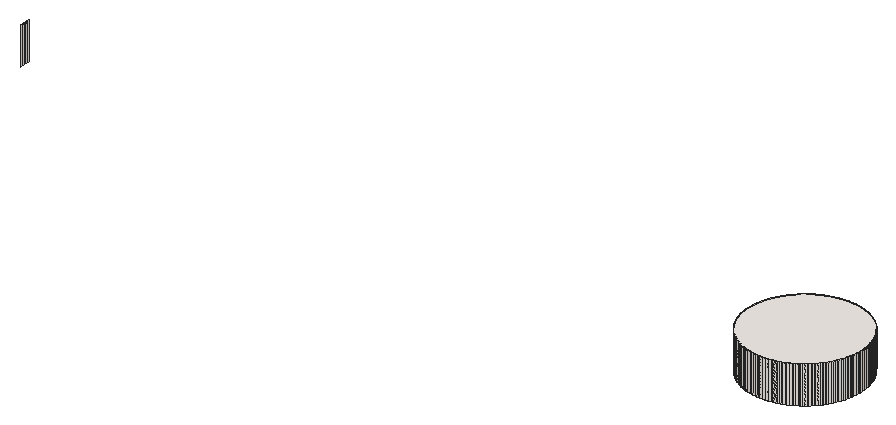
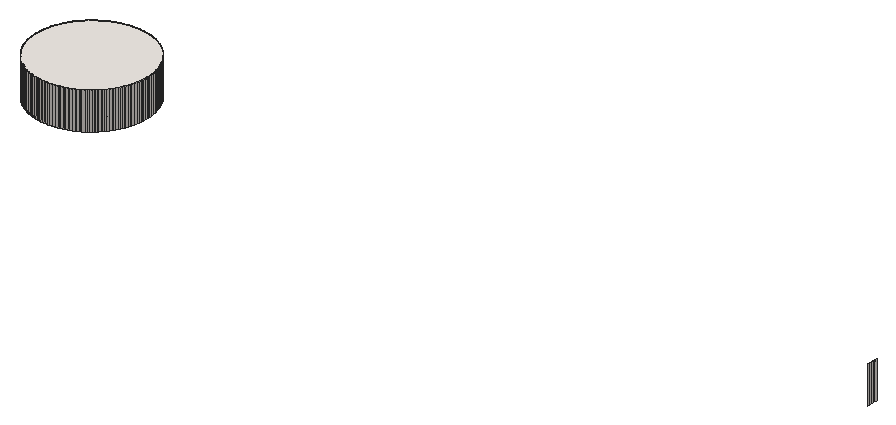
# SketchUp Ruby script. Lengths in inches.
U = 1.inch
M = Sketchup.active_model
def pt(a) = Geom::Point3d.new(a.map { |v| v * U })
def face(e, loops, mat)
  f = e.add_face(loops[0].map { |a| pt(a) })
  loops[1..].each { |l| e.add_face(l.map { |a| pt(a) }).erase! }
  f.material = f.back_material = mat if mat
  f
end
# faces: each face lists its corners as indices into pts; further lists are holes
def faces(e, pts, list, mat = nil) = list.each { |f| face(e, (f[0].is_a?(Array) ? f : [f]).map { |l| l.map { |i| pts[i] } }, mat) }
# xy, xz, yz: faces in a plane at the given z, y or x. An outline is a flat list of corners, or four numbers for a rectangle; further outlines are holes
def ring(l) = l.size == 4 ? [[l[0], l[1]], [l[2], l[1]], [l[2], l[3]], [l[0], l[3]]] : l.each_slice(2).to_a
def flat(e, list, mat, &to3) = list.each { |f| face(e, (f[0].is_a?(Array) ? f : [f]).map { |l| ring(l).map { |u, v| to3.(u, v) } }, mat) }
def xy(e, z, list, mat = nil) = flat(e, list, mat) { |x, y| [x, y, z] }
def xz(e, y, list, mat = nil) = flat(e, list, mat) { |x, z| [x, y, z] }
def yz(e, x, list, mat = nil) = flat(e, list, mat) { |y, z| [x, y, z] }
def lines(e, pts, list) = list.each { |a, b| e.add_line(pt(pts[a]), pt(pts[b])) }
# prism: a flat outline (further loops are holes) pulled along v
def prism(e, loops, v, mat = nil)
  f = face(e, loops, mat); d = Geom::Vector3d.new(v.map { |x| x * U })
  f.pushpull(f.normal.samedirection?(d) ? d.length : -d.length)
end
def box(e, o, s, mat = nil) = prism(e, [[o, [o[0] + s[0], o[1], o[2]], [o[0] + s[0], o[1] + s[1], o[2]], [o[0], o[1] + s[1], o[2]]]], [0, 0, s[2]], mat)
def at(x, y, z, deg = 0) = Geom::Transformation.translation(pt([x, y, z])) * Geom::Transformation.rotation(ORIGIN, Z_AXIS, deg.degrees)
def axes(o, x, y, z) = Geom::Transformation.new([*x, 0, *y, 0, *z, 0, *pt(o).to_a, 1])
def part(name) = M.definitions.add(name)
# library, detail: a bought-in or finely detailed component or shape, given as its bounding box
def library(name, o, s) = part(name).tap { |d| box(d.entities, o, s) }
def detail(e, o, s) = box(e.add_group.entities, o, s)
def put(e, d, t, mat = nil) = e.add_instance(d, t).tap { |i| i.material = mat if mat }
def group(e, t, mat = nil) = e.add_group.tap { |g| g.transformation = t; g.material = mat if mat }.entities
root = M.entities
M.materials.add("0001 AP 9436 AIR BREEZE").color = [243, 237, 232]
xy(root,108,[[158.91,40.5,158.83,40.51,158.75,40.51,158.51,40.54,158.4375,40.55,158.36,40.57,158.28,40.59,158.21,40.61,158.13,40.63,158.06,40.65,157.98,40.68,157.91,40.71,157.84,40.73,157.76,40.77,157.69,40.8,157.625,40.83,157.55,40.87,157.49,40.91,157.35,40.99,157.29,41.04,157.22,41.08,156.98,41.28,156.87,41.39,156.8125,41.45,156.76,41.5,156.61,41.6875,156.5625,41.75,156.52,41.8125,156.48,41.88,156.43,41.95,156.39,42.01,156.36,42.08,156.32,42.15,156.29,42.22,156.25,42.29,156.22,42.37,156.19,42.44,156.17,42.51,156.14,42.59,156.12,42.66,156.0625,42.89,156.05,42.97,156.03,43.05,156.01,43.2,156.01,43.28,156,43.36,156,43.59,156.01,43.67,156.01,43.75,156.04,43.99,156.05,44.0625,156.07,44.14,156.09,44.22,156.11,44.29,156.13,44.37,156.15,44.44,156.18,44.52,156.21,44.59,156.23,44.66,156.27,44.74,156.3,44.81,156.33,44.875,156.37,44.95,156.41,45.01,156.49,45.15,156.54,45.21,156.58,45.28,156.78,45.52,156.89,45.63,156.95,45.6875,157,45.74,157.1875,45.89,157.25,45.9375,157.3125,45.98,157.38,46.02,157.45,46.07,157.51,46.11,157.58,46.14,157.65,46.18,157.72,46.21,157.79,46.25,157.87,46.28,157.94,46.31,158.01,46.33,158.09,46.36,158.16,46.38,158.39,46.4375,158.47,46.45,158.55,46.47,158.7,46.49,158.78,46.49,158.86,46.5,159.09,46.5,159.17,46.49,159.25,46.49,159.49,46.46,159.5625,46.45,159.64,46.43,159.72,46.41,159.79,46.39,159.87,46.37,159.94,46.35,160.02,46.32,160.09,46.29,160.16,46.27,160.24,46.23,160.31,46.2,160.375,46.17,160.45,46.13,160.51,46.09,160.65,46.01,160.71,45.96,160.78,45.92,161.02,45.72,161.13,45.61,161.1875,45.55,161.24,45.5,161.39,45.3125,161.4375,45.25,161.48,45.1875,161.52,45.12,161.57,45.05,161.61,44.99,161.64,44.92,161.68,44.85,161.71,44.78,161.75,44.71,161.78,44.63,161.81,44.56,161.83,44.49,161.86,44.41,161.88,44.34,161.9375,44.11,161.95,44.03,161.97,43.95,161.99,43.8,161.99,43.72,162,43.64,162,43.41,161.99,43.33,161.99,43.25,161.96,43.01,161.95,42.9375,161.93,42.86,161.91,42.78,161.89,42.71,161.87,42.63,161.85,42.56,161.82,42.48,161.79,42.41,161.77,42.34,161.73,42.26,161.7,42.19,161.67,42.125,161.63,42.05,161.59,41.99,161.51,41.85,161.46,41.79,161.42,41.72,161.22,41.48,161.11,41.37,161.05,41.3125,161,41.26,160.8125,41.11,160.75,41.0625,160.6875,41.02,160.62,40.98,160.55,40.93,160.49,40.89,160.42,40.86,160.35,40.82,160.28,40.79,160.21,40.75,160.13,40.72,160.06,40.69,159.99,40.67,159.91,40.64,159.84,40.62,159.61,40.5625,159.53,40.55,159.45,40.53,159.3,40.51,159.22,40.51,159.14,40.5]],"0001 AP 9436 AIR BREEZE")
xz(root,40.5,[[158.91,106,158.98,108],[158.98,106,159.0625,108],[159.0625,106,159.14,108]],"0001 AP 9436 AIR BREEZE")
xz(root,40.51,[[158.75,106,158.83,108],[159.22,106,159.3,108]],"0001 AP 9436 AIR BREEZE")
xz(root,46.49,[[158.7,106,158.78,108],[159.17,106,159.25,108]],"0001 AP 9436 AIR BREEZE")
xz(root,46.5,[[158.86,106,158.9375,108],[158.9375,106,159.02,108],[159.02,106,159.09,108]],"0001 AP 9436 AIR BREEZE")
yz(root,116.99,[[43.25,106,43.33,108],[43.72,106,43.8,108]],"0001 AP 9436 AIR BREEZE")
yz(root,117,[[43.41,106,43.48,108],[43.48,106,43.5625,108],[43.5625,106,43.64,108]],"0001 AP 9436 AIR BREEZE")
yz(root,156,[[43.36,106,43.4375,108],[43.4375,106,43.52,108],[43.52,106,43.59,108]],"0001 AP 9436 AIR BREEZE")
yz(root,156.01,[[43.2,106,43.28,108],[43.67,106,43.75,108]],"0001 AP 9436 AIR BREEZE")
yz(root,161.99,[[43.25,106,43.33,108],[43.72,106,43.8,108]],"0001 AP 9436 AIR BREEZE")
yz(root,162,[[43.41,106,43.48,108],[43.48,106,43.5625,108],[43.5625,106,43.64,108]],"0001 AP 9436 AIR BREEZE")
p = [[158.51,40.54,106],[158.4375,40.55,106],[158.4375,40.55,108],[158.51,40.54,108],[158.59,40.53,106],[158.59,40.53,108],
  [158.67,40.52,106],[158.67,40.52,108],[158.75,40.51,106],[158.75,40.51,108],[158.91,40.5,106],[158.83,40.51,106],
  [158.83,40.51,108],[158.91,40.5,108],[159.22,40.51,106],[159.14,40.5,106],[159.14,40.5,108],[159.22,40.51,108],
  [159.375,40.52,106],[159.3,40.51,106],[159.3,40.51,108],[159.375,40.52,108],[159.45,40.53,106],[159.45,40.53,108],
  [159.53,40.55,106],[159.53,40.55,108],[159.61,40.5625,106],[159.61,40.5625,108],[158.13,40.63,106],[158.06,40.65,106],
  [158.06,40.65,108],[158.13,40.63,108],[158.21,40.61,106],[158.21,40.61,108],[158.28,40.59,106],[158.28,40.59,108],
  [158.36,40.57,106],[158.36,40.57,108],[159.68,40.58,106],[159.68,40.58,108],[159.76,40.6,106],[159.76,40.6,108],
  [159.84,40.62,106],[159.84,40.62,108],[159.91,40.64,106],[159.91,40.64,108],[159.99,40.67,106],[159.99,40.67,108],
  [157.84,40.73,106],[157.76,40.77,106],[157.76,40.77,108],[157.84,40.73,108],[157.91,40.71,106],[157.91,40.71,108],
  [157.98,40.68,106],[157.98,40.68,108],[160.06,40.69,106],[160.06,40.69,108],[160.13,40.72,106],[160.13,40.72,108],
  [160.21,40.75,106],[160.21,40.75,108],[157.625,40.83,106],[157.55,40.87,106],[157.55,40.87,108],[157.625,40.83,108],
  [157.69,40.8,106],[157.69,40.8,108],[160.28,40.79,106],[160.28,40.79,108],[160.35,40.82,106],[160.35,40.82,108],
  [160.42,40.86,106],[160.42,40.86,108],[157.49,40.91,106],[157.42,40.95,106],[157.42,40.95,108],[157.49,40.91,108],
  [160.49,40.89,106],[160.49,40.89,108],[160.55,40.93,106],[160.55,40.93,108],[160.62,40.98,106],[160.62,40.98,108],
  [157.29,41.04,106],[157.22,41.08,106],[157.22,41.08,108],[157.29,41.04,108],[157.35,40.99,106],[157.35,40.99,108],
  [160.6875,41.02,106],[160.6875,41.02,108],[160.75,41.0625,106],[160.75,41.0625,108],[157.16,41.13,106],[157.1,41.18,106],
  [157.1,41.18,108],[157.16,41.13,108],[160.8125,41.11,106],[160.8125,41.11,108],[160.875,41.16,106],[160.875,41.16,108],
  [157.04,41.23,106],[156.98,41.28,106],[156.98,41.28,108],[157.04,41.23,108],[160.9375,41.21,106],[160.9375,41.21,108],
  [161,41.26,106],[161,41.26,108],[156.92,41.34,106],[156.87,41.39,106],[156.87,41.39,108],[156.92,41.34,108],
  [161.05,41.3125,106],[161.05,41.3125,108],[161.11,41.37,106],[161.11,41.37,108],[156.8125,41.45,106],[156.76,41.5,106],
  [156.76,41.5,108],[156.8125,41.45,108],[161.16,41.42,106],[161.16,41.42,108],[161.22,41.48,106],[161.22,41.48,108],
  [156.71,41.5625,106],[156.71,41.5625,108],[161.27,41.54,106],[161.27,41.54,108],[161.32,41.6,106],[161.32,41.6,108],
  [156.66,41.625,106],[156.61,41.6875,106],[156.61,41.6875,108],[156.66,41.625,108],[161.37,41.66,106],[161.37,41.66,108],
  [156.5625,41.75,106],[156.52,41.8125,106],[156.52,41.8125,108],[156.5625,41.75,108],[161.42,41.72,106],[161.42,41.72,108],
  [161.46,41.79,106],[161.46,41.79,108],[156.48,41.88,106],[156.48,41.88,108],[161.51,41.85,106],[161.51,41.85,108],
  [156.43,41.95,106],[156.39,42.01,106],[156.39,42.01,108],[156.43,41.95,108],[161.55,41.92,106],[161.55,41.92,108],
  [161.59,41.99,106],[161.59,41.99,108],[156.36,42.08,106],[156.36,42.08,108],[161.63,42.05,106],[161.63,42.05,108],
  [156.32,42.15,106],[156.32,42.15,108],[161.67,42.125,106],[161.67,42.125,108],[161.7,42.19,106],[161.7,42.19,108],
  [156.29,42.22,106],[156.25,42.29,106],[156.25,42.29,108],[156.29,42.22,108],[161.73,42.26,106],[161.73,42.26,108],
  [156.22,42.37,106],[156.22,42.37,108],[161.77,42.34,106],[161.77,42.34,108],[161.79,42.41,106],[161.79,42.41,108],
  [156.19,42.44,106],[156.17,42.51,106],[156.17,42.51,108],[156.19,42.44,108],[161.82,42.48,106],[161.82,42.48,108],
  [156.14,42.59,106],[156.14,42.59,108],[161.85,42.56,106],[161.85,42.56,108],[156.12,42.66,106],[156.12,42.66,108],
  [161.87,42.63,106],[161.87,42.63,108],[161.89,42.71,106],[161.89,42.71,108],[156.1,42.74,106],[156.08,42.82,106],
  [156.08,42.82,108],[156.1,42.74,108],[161.91,42.78,106],[161.91,42.78,108],[156.0625,42.89,106],[156.0625,42.89,108],
  [161.93,42.86,106],[161.93,42.86,108],[156.05,42.97,106],[156.05,42.97,108],[161.95,42.9375,106],[161.95,42.9375,108],
  [161.96,43.01,106],[161.96,43.01,108],[156.03,43.05,106],[156.02,43.125,106],[156.02,43.125,108],[156.03,43.05,108],
  [161.97,43.09,106],[161.97,43.09,108],[156.01,43.2,106],[156.01,43.2,108],[161.98,43.17,106],[161.98,43.17,108],
  [161.99,43.25,106],[161.99,43.25,108],[117,43.41,106],[116.99,43.33,106],[116.99,43.33,108],[117,43.41,108],
  [156.01,43.28,106],[156,43.36,106],[156,43.36,108],[156.01,43.28,108],[162,43.41,106],[161.99,43.33,106],
  [161.99,43.33,108],[162,43.41,108],[116.99,43.72,106],[117,43.64,106],[117,43.64,108],[116.99,43.72,108],
  [156,43.59,106],[156.01,43.67,106],[156.01,43.67,108],[156,43.59,108],[161.99,43.72,106],[162,43.64,106],
  [162,43.64,108],[161.99,43.72,108],[156.01,43.75,106],[156.02,43.83,106],[156.02,43.83,108],[156.01,43.75,108],
  [156.03,43.91,106],[156.03,43.91,108],[161.98,43.875,106],[161.99,43.8,106],[161.99,43.8,108],[161.98,43.875,108],
  [156.04,43.99,106],[156.04,43.99,108],[161.97,43.95,106],[161.97,43.95,108],[156.05,44.0625,106],[156.05,44.0625,108],
  [161.9375,44.11,106],[161.95,44.03,106],[161.95,44.03,108],[161.9375,44.11,108],[156.07,44.14,106],[156.07,44.14,108],
  [156.09,44.22,106],[156.09,44.22,108],[161.92,44.18,106],[161.92,44.18,108],[156.11,44.29,106],[156.11,44.29,108],
  [161.9,44.26,106],[161.9,44.26,108],[156.13,44.37,106],[156.13,44.37,108],[161.86,44.41,106],[161.88,44.34,106],
  [161.88,44.34,108],[161.86,44.41,108],[156.15,44.44,106],[156.15,44.44,108],[156.18,44.52,106],[156.18,44.52,108],
  [161.83,44.49,106],[161.83,44.49,108],[156.21,44.59,106],[156.21,44.59,108],[161.81,44.56,106],[161.81,44.56,108],
  [156.23,44.66,106],[156.23,44.66,108],[161.75,44.71,106],[161.78,44.63,106],[161.78,44.63,108],[161.75,44.71,108],
  [156.27,44.74,106],[156.27,44.74,108],[156.3,44.81,106],[156.3,44.81,108],[161.71,44.78,106],[161.71,44.78,108],
  [156.33,44.875,106],[156.33,44.875,108],[161.64,44.92,106],[161.68,44.85,106],[161.68,44.85,108],[161.64,44.92,108],
  [156.37,44.95,106],[156.37,44.95,108],[156.41,45.01,106],[156.41,45.01,108],[161.61,44.99,106],[161.61,44.99,108],
  [156.45,45.08,106],[156.45,45.08,108],[161.57,45.05,106],[161.57,45.05,108],[156.49,45.15,106],[156.49,45.15,108],
  [156.54,45.21,106],[156.54,45.21,108],[161.48,45.1875,106],[161.52,45.12,106],[161.52,45.12,108],[161.48,45.1875,108],
  [156.58,45.28,106],[156.58,45.28,108],[161.4375,45.25,106],[161.4375,45.25,108],[156.63,45.34,106],[156.63,45.34,108],
  [156.68,45.4,106],[156.68,45.4,108],[161.34,45.375,106],[161.39,45.3125,106],[161.39,45.3125,108],[161.34,45.375,108],
  [156.73,45.46,106],[156.73,45.46,108],[161.24,45.5,106],[161.29,45.4375,106],[161.29,45.4375,108],[161.24,45.5,108],
  [156.78,45.52,106],[156.78,45.52,108],[156.84,45.58,106],[156.84,45.58,108],[161.1875,45.55,106],[161.1875,45.55,108],
  [156.89,45.63,106],[156.89,45.63,108],[156.95,45.6875,106],[156.95,45.6875,108],[161.08,45.66,106],[161.13,45.61,106],
  [161.13,45.61,108],[161.08,45.66,108],[157,45.74,106],[157,45.74,108],[157.0625,45.79,106],[157.0625,45.79,108],
  [160.96,45.77,106],[161.02,45.72,106],[161.02,45.72,108],[160.96,45.77,108],[157.125,45.84,106],[157.125,45.84,108],
  [157.1875,45.89,106],[157.1875,45.89,108],[160.84,45.87,106],[160.9,45.82,106],[160.9,45.82,108],[160.84,45.87,108],
  [157.25,45.9375,106],[157.25,45.9375,108],[157.3125,45.98,106],[157.3125,45.98,108],[160.71,45.96,106],[160.78,45.92,106],
  [160.78,45.92,108],[160.71,45.96,108],[157.38,46.02,106],[157.38,46.02,108],[157.45,46.07,106],[157.45,46.07,108],
  [160.51,46.09,106],[160.58,46.05,106],[160.58,46.05,108],[160.51,46.09,108],[160.65,46.01,106],[160.65,46.01,108],
  [157.51,46.11,106],[157.51,46.11,108],[157.58,46.14,106],[157.58,46.14,108],[157.65,46.18,106],[157.65,46.18,108],
  [160.375,46.17,106],[160.45,46.13,106],[160.45,46.13,108],[160.375,46.17,108],[157.72,46.21,106],[157.72,46.21,108],
  [157.79,46.25,106],[157.79,46.25,108],[157.87,46.28,106],[157.87,46.28,108],[160.16,46.27,106],[160.24,46.23,106],
  [160.24,46.23,108],[160.16,46.27,108],[160.31,46.2,106],[160.31,46.2,108],[157.94,46.31,106],[157.94,46.31,108],
  [158.01,46.33,106],[158.01,46.33,108],[158.09,46.36,106],[158.09,46.36,108],[159.87,46.37,106],[159.94,46.35,106],
  [159.94,46.35,108],[159.87,46.37,108],[160.02,46.32,106],[160.02,46.32,108],[160.09,46.29,106],[160.09,46.29,108],
  [158.16,46.38,106],[158.16,46.38,108],[158.24,46.4,106],[158.24,46.4,108],[158.32,46.42,106],[158.32,46.42,108],
  [158.39,46.4375,106],[158.39,46.4375,108],[158.47,46.45,106],[158.47,46.45,108],[159.49,46.46,106],[159.5625,46.45,106],
  [159.5625,46.45,108],[159.49,46.46,108],[159.64,46.43,106],[159.64,46.43,108],[159.72,46.41,106],[159.72,46.41,108],
  [159.79,46.39,106],[159.79,46.39,108],[158.55,46.47,106],[158.55,46.47,108],[158.625,46.48,106],[158.625,46.48,108],
  [158.7,46.49,106],[158.7,46.49,108],[158.78,46.49,106],[158.86,46.5,106],[158.86,46.5,108],[158.78,46.49,108],
  [159.09,46.5,106],[159.17,46.49,106],[159.17,46.49,108],[159.09,46.5,108],[159.25,46.49,106],[159.33,46.48,106],
  [159.33,46.48,108],[159.25,46.49,108],[159.41,46.47,106],[159.41,46.47,108]]
faces(root,p,[[0,1,2,3],[4,0,3,5],[6,4,5,7],[8,6,7,9],[10,11,12,13],[14,15,16,17],[18,19,20,21],[22,18,21,23],
  [24,22,23,25],[26,24,25,27],[28,29,30,31],[32,28,31,33],[34,32,33,35],[36,34,35,37],[1,36,37,2],[38,26,27,39],
  [40,38,39,41],[42,40,41,43],[44,42,43,45],[46,44,45,47],[48,49,50,51],[52,48,51,53],[54,52,53,55],[29,54,55,30],
  [56,46,47,57],[58,56,57,59],[60,58,59,61],[62,63,64,65],[66,62,65,67],[49,66,67,50],[68,60,61,69],[70,68,69,71],
  [72,70,71,73],[74,75,76,77],[63,74,77,64],[78,72,73,79],[80,78,79,81],[82,80,81,83],[84,85,86,87],[88,84,87,89],
  [75,88,89,76],[90,82,83,91],[92,90,91,93],[94,95,96,97],[85,94,97,86],[98,92,93,99],[100,98,99,101],[102,103,104,105],
  [95,102,105,96],[106,100,101,107],[108,106,107,109],[110,111,112,113],[103,110,113,104],[114,108,109,115],[116,114,115,117],[118,119,120,121],
  [111,118,121,112],[122,116,117,123],[124,122,123,125],[119,126,127,120],[128,124,125,129],[130,128,129,131],[132,133,134,135],[126,132,135,127],
  [136,130,131,137],[138,139,140,141],[133,138,141,134],[142,136,137,143],[144,142,143,145],[139,146,147,140],[148,144,145,149],[150,151,152,153],
  [146,150,153,147],[154,148,149,155],[156,154,155,157],[151,158,159,152],[160,156,157,161],[158,162,163,159],[164,160,161,165],[166,164,165,167],
  [168,169,170,171],[162,168,171,163],[172,166,167,173],[169,174,175,170],[176,172,173,177],[178,176,177,179],[180,181,182,183],[174,180,183,175],
  [184,178,179,185],[181,186,187,182],[188,184,185,189],[186,190,191,187],[192,188,189,193],[194,192,193,195],[196,197,198,199],[190,196,199,191],
  [200,194,195,201],[197,202,203,198],[204,200,201,205],[202,206,207,203],[208,204,205,209],[210,208,209,211],[212,213,214,215],[206,212,215,207],
  [216,210,211,217],[213,218,219,214],[220,216,217,221],[222,220,221,223],[224,225,226,227],[228,229,230,231],[232,233,234,235],[236,237,238,239],
  [240,241,242,243],[244,245,246,247],[248,249,250,251],[249,252,253,250],[254,255,256,257],[252,258,259,253],[260,254,257,261],[258,262,263,259],
  [264,265,266,267],[265,260,261,266],[262,268,269,263],[268,270,271,269],[272,264,267,273],[270,274,275,271],[276,272,273,277],[274,278,279,275],
  [280,281,282,283],[281,276,277,282],[278,284,285,279],[284,286,287,285],[288,280,283,289],[286,290,291,287],[292,288,289,293],[290,294,295,291],
  [296,297,298,299],[297,292,293,298],[294,300,301,295],[300,302,303,301],[304,296,299,305],[302,306,307,303],[308,309,310,311],[309,304,305,310],
  [306,312,313,307],[312,314,315,313],[316,308,311,317],[314,318,319,315],[320,316,317,321],[318,322,323,319],[322,324,325,323],[326,327,328,329],
  [327,320,321,328],[324,330,331,325],[332,326,329,333],[330,334,335,331],[334,336,337,335],[338,339,340,341],[339,332,333,340],[336,342,343,337],
  [344,345,346,347],[345,338,341,346],[342,348,349,343],[348,350,351,349],[352,344,347,353],[350,354,355,351],[354,356,357,355],[358,359,360,361],
  [359,352,353,360],[356,362,363,357],[362,364,365,363],[366,367,368,369],[367,358,361,368],[364,370,371,365],[370,372,373,371],[374,375,376,377],
  [375,366,369,376],[372,378,379,373],[378,380,381,379],[382,383,384,385],[383,374,377,384],[380,386,387,381],[386,388,389,387],[390,391,392,393],
  [391,394,395,392],[394,382,385,395],[388,396,397,389],[396,398,399,397],[398,400,401,399],[402,403,404,405],[403,390,393,404],[400,406,407,401],
  [406,408,409,407],[408,410,411,409],[412,413,414,415],[413,416,417,414],[416,402,405,417],[410,418,419,411],[418,420,421,419],[420,422,423,421],
  [424,425,426,427],[425,428,429,426],[428,430,431,429],[430,412,415,431],[422,432,433,423],[432,434,435,433],[434,436,437,435],[436,438,439,437],
  [438,440,441,439],[442,443,444,445],[443,446,447,444],[446,448,449,447],[448,450,451,449],[450,424,427,451],[440,452,453,441],[452,454,455,453],
  [454,456,457,455],[458,459,460,461],[462,463,464,465],[466,467,468,469],[467,470,471,468],[470,442,445,471]],"0001 AP 9436 AIR BREEZE")
